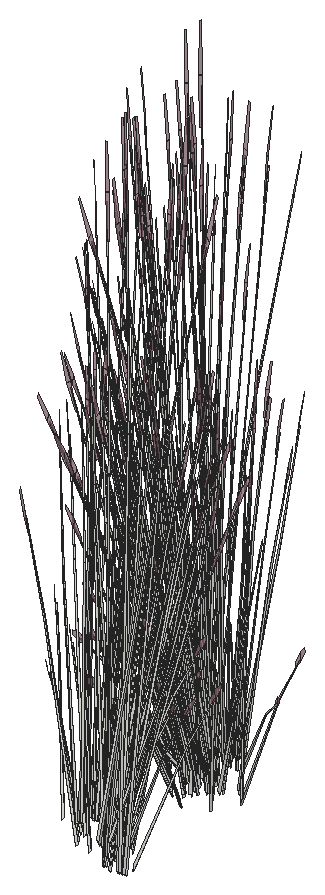
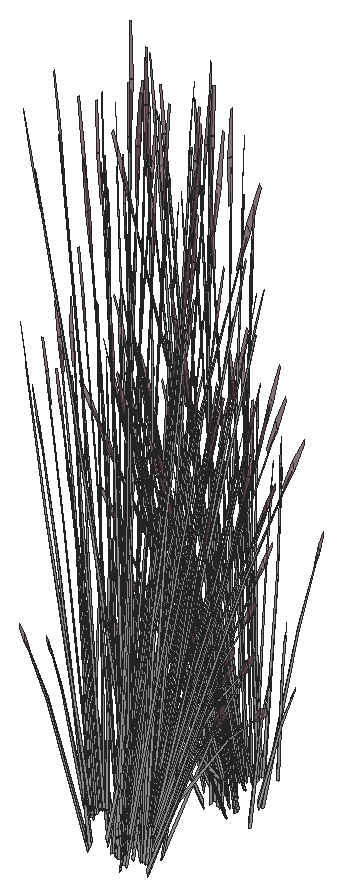
# SketchUp Ruby script. Lengths in inches.
U = 1.inch
M = Sketchup.active_model
def pt(a) = Geom::Point3d.new(a.map { |v| v * U })
def face(e, loops, mat)
  f = e.add_face(loops[0].map { |a| pt(a) })
  loops[1..].each { |l| e.add_face(l.map { |a| pt(a) }).erase! }
  f.material = f.back_material = mat if mat
  f
end
# faces: each face lists its corners as indices into pts; further lists are holes
def faces(e, pts, list, mat = nil) = list.each { |f| face(e, (f[0].is_a?(Array) ? f : [f]).map { |l| l.map { |i| pts[i] } }, mat) }
# xy, xz, yz: faces in a plane at the given z, y or x. An outline is a flat list of corners, or four numbers for a rectangle; further outlines are holes
def ring(l) = l.size == 4 ? [[l[0], l[1]], [l[2], l[1]], [l[2], l[3]], [l[0], l[3]]] : l.each_slice(2).to_a
def flat(e, list, mat, &to3) = list.each { |f| face(e, (f[0].is_a?(Array) ? f : [f]).map { |l| ring(l).map { |u, v| to3.(u, v) } }, mat) }
def xy(e, z, list, mat = nil) = flat(e, list, mat) { |x, y| [x, y, z] }
def xz(e, y, list, mat = nil) = flat(e, list, mat) { |x, z| [x, y, z] }
def yz(e, x, list, mat = nil) = flat(e, list, mat) { |y, z| [x, y, z] }
def lines(e, pts, list) = list.each { |a, b| e.add_line(pt(pts[a]), pt(pts[b])) }
# prism: a flat outline (further loops are holes) pulled along v
def prism(e, loops, v, mat = nil)
  f = face(e, loops, mat); d = Geom::Vector3d.new(v.map { |x| x * U })
  f.pushpull(f.normal.samedirection?(d) ? d.length : -d.length)
end
def box(e, o, s, mat = nil) = prism(e, [[o, [o[0] + s[0], o[1], o[2]], [o[0] + s[0], o[1] + s[1], o[2]], [o[0], o[1] + s[1], o[2]]]], [0, 0, s[2]], mat)
def at(x, y, z, deg = 0) = Geom::Transformation.translation(pt([x, y, z])) * Geom::Transformation.rotation(ORIGIN, Z_AXIS, deg.degrees)
def axes(o, x, y, z) = Geom::Transformation.new([*x, 0, *y, 0, *z, 0, *pt(o).to_a, 1])
def part(name) = M.definitions.add(name)
# library, detail: a bought-in or finely detailed component or shape, given as its bounding box
def library(name, o, s) = part(name).tap { |d| box(d.entities, o, s) }
def detail(e, o, s) = box(e.add_group.entities, o, s)
def put(e, d, t, mat = nil) = e.add_instance(d, t).tap { |i| i.material = mat if mat }
def group(e, t, mat = nil) = e.add_group.tap { |g| g.transformation = t; g.material = mat if mat }.entities
root = M.entities
M.materials.add("LightPink_Translucent").color = [144, 107, 117]
M.materials["LightPink_Translucent"].alpha = 0.75
c1 = part("blade")
p = [[2.15,0.21,22],[0,0.17,0],[0.09,0.45,0],[2.18,0.31,22],[2.29,0.31,22],[0.38,0.45,0],
  [2.48,0.24,33],[2.49,0.24,33],[2.48,0.22,33]]
faces(c1.entities,p,[[0,1,2,3],[4,5,2,3],[6,3,4,7],[8,0,3,6]])
c2 = part("seeds")
p = [[0.3,-0.1,1.38],[-0.01,-0.03,1.59],[-0.01,-0.03,0.03],[0.14,-0.07,-0.07],[0.29,-0.03,3],[0.15,0.01,3.11]]
faces(c2.entities,p,[[0,1,2,3],[1,0,4,5]],"LightPink_Translucent")
c3 = part("blade with seeds")
put(c3.entities,c1,at(0,0,0))
put(c3.entities,c2,axes([2.4,0.25,30.99],[1.5799,-0.05474,1.17369],[-0.12525,1.92788,0.29478],[-0.07173,-0.02425,1.56792]))
put(root,c3,axes([417.64,637.87,155.99],[-0.38233,-0.1167,-0.2617],[0.09626,-0.41098,0.2617],[-0.07708,0.04739,1.17405]))
put(root,c3,axes([414.88,637.03,156.46],[0.14242,0.03872,1.20808],[0.09179,0.39548,-0.25981],[-0.19345,0.07403,0.51652]))
put(root,c3,axes([415.52,636.71,158.54],[0.35672,-0.06741,0.29918],[0.09419,0.38534,-0.38624],[-0.10222,0.1035,0.73904]))
put(root,c3,axes([419.12,636.3,156.28],[0.51243,0,0],[0,0.52715,-0.43598],[0,0.12006,1.38303]))
put(root,c3,axes([414.14,636.54,158.25],[0.0523,0.01265,1.49853],[0.16179,0.41674,-0.1416],[-0.10706,0.10938,0.26519]))
put(root,c3,axes([418.91,636.57,156.13],[-0.51218,-0.00377,-0.04204],[0,-0.52715,0.42192],[-0.0161,0.12,1.33776]))
put(root,c3,axes([417.8,636.11,156.53],[0.46151,0.22505,-0.2458],[-0.22222,0.475,-0.42242],[0.0145,0.11662,1.34921]))
put(root,c3,axes([414.58,637.86,156.61],[0.17079,-0.21377,0.97034],[0.06739,0.33841,0.71294],[-0.12342,0.0606,0.21373]))
put(root,c3,axes([418.69,637.47,158.1],[0.23317,0.29531,-0.29918],[-0.26625,0.27955,0.38624],[0.13527,0.04253,0.73904]))
put(root,c3,axes([418.8,636.65,155.99],[-0.28606,0.29428,-0.2617],[-0.28606,-0.29428,0.2617],[0,0.09479,1.17405]))
put(root,c3,axes([417.57,636.68,156.53],[0.04775,0.53819,-0.2458],[-0.49736,0.03254,-0.42242],[-0.08758,0.07169,1.34921]))
put(root,c3,axes([418.57,637.58,158.27],[-0.02064,0.35866,0.05432],[-0.3116,-0.00983,0.42765],[0.11936,0.03753,0.65209]))
put(root,c3,axes([417.75,636.47,156.14],[-0.19883,0.425,-0.37796],[-0.41314,-0.20454,0.1819],[0,0.09797,1.2135]))
put(root,c3,axes([415.23,636.9375,158.1],[-0.35672,0.06741,-0.29918],[-0.09419,-0.38534,0.38624],[-0.10222,0.1035,0.73904]))
put(root,c3,axes([418.6,637.47,158.27],[-0.30217,0.31079,0.40553],[-0.2606,-0.33005,0.33437],[0.14177,0.05733,0.83914]))
put(root,c3,axes([414.71,637.8,159.05],[0.36162,0.1259,-0.05481],[-0.11124,0.3875,-0.2485],[-0.05915,0.05883,0.81966]))
put(root,c3,axes([417.27,637.09,156.02],[-0.27603,0.35451,-0.52676],[-0.34289,-0.32147,-0.13825],[-0.11061,0.08844,1.16273]))
put(root,c3,axes([417.64,637.83,158.54],[-0.06329,-0.37991,0.29918],[0.36182,-0.10032,-0.38624],[0.09718,0.10887,0.73904]))
put(root,c3,axes([417.76,637.68,156.24],[0.51304,0.1533,0.25983],[-0.12835,0.54797,-0.30828],[-0.08491,0.06858,1.39295]))
put(root,c3,axes([417.73,638.05,155.98],[-0.38354,0.23583,-0.41945],[-0.22925,-0.42288,0],[-0.08735,0.05371,1.33059]))
put(root,c3,axes([419,636.66,155.98],[0,0.47166,-0.41945],[-0.45849,0,0],[0,0.10742,1.33059]))
put(root,c3,axes([417.86,636.71,157.55],[-0.15222,-0.08126,1.44779],[0.31502,-0.34091,0.11706],[0.19634,0.15379,0.61892]))
put(root,c3,axes([417.88,635.64,158.06],[-0.35411,-0.24507,1.16821],[0.37391,-0.38156,0.50405],[0.11425,0.22994,1.12919]))
put(root,c3,axes([415.33,636.68,158.53],[0.37908,0.26007,-0.10273],[-0.21839,0.37663,-0.57019],[-0.1071,0.13092,0.8664]))
put(root,c3,axes([418.42,637.64,156.61],[-0.23074,-0.13562,0.97034],[0.29794,-0.1378,0.71294],[0.08036,0.11673,0.21373]))
put(root,c3,axes([417.61,638.02,158.53],[0.2442,-0.40372,-0.10273],[0.35364,0.23259,-0.57019],[0.12293,0.11406,0.8664]))
put(root,c3,axes([415.84,636.56,157.55],[0.10236,-0.14492,1.44779],[0.25844,0.39118,0.11706],[-0.17726,0.17814,0.61892]))
put(root,c3,axes([415.52,636.98,158.23],[0.10528,0.43067,-0.43168],[-0.39868,0.07534,-0.33437],[-0.11425,0.11568,0.82598]))
put(root,c3,axes([416,637.48,158.54],[0.27728,-0.24833,0.29918],[0.26248,0.28355,-0.38624],[-0.03994,0.14407,0.73904]))
put(root,c3,axes([418.08,637.98,156.28],[0.25622,0.47263,0],[-0.42866,0.26357,-0.43598],[-0.09763,0.06003,1.38303]))
put(root,c3,axes([417.29,638.36,158.25],[0.00121,-0.0571,1.49853],[0.35119,-0.25193,-0.1416],[0.12199,0.08992,0.26519]))
put(root,c3,axes([418.48,638.14,155.54],[0.02986,-0.06809,1.48974],[0.37589,-0.20055,-0.22758],[0.11396,0.1038,0.25375]))
put(root,c3,axes([417.86,636.11,156.68],[-0.01119,-0.44408,1.19347],[0.50665,0.11511,0.50532],[-0.11983,0.243,1.12654]))
put(root,c3,axes([417.99,636.59,156.05],[0.15027,0.43184,-0.5847],[-0.43285,0.15553,-0.15346],[0.01661,0.14623,1.29063]))
put(root,c3,axes([415.75,637.7,158.27],[-0.33677,-0.02198,0.05432],[0.00923,-0.33185,0.42765],[-0.03524,0.12712,0.65209]))
put(root,c3,axes([415.03,638.08,155.54],[0.05497,0.04712,1.48974],[0.09321,0.43661,-0.22758],[-0.12183,0.0931,0.25375]))
put(root,c3,axes([415.85,637.73,158.27],[-0.29182,-0.32181,0.40553],[0.3099,-0.27755,0.33437],[-0.05383,0.15098,0.83914]))
put(root,c3,axes([417.9,637.82,158.23],[0.40438,-0.11212,-0.43168],[0.07074,0.4246,-0.33437],[0.10862,0.12168,0.82598]))
put(root,c3,axes([416.78,637.89,158.54],[0.12355,-0.36271,0.29918],[0.36044,0.10579,-0.38624],[0.03305,0.14603,0.73904]))
put(root,c3,axes([418.46,638.25,156.53],[-0.26279,-0.01479,0.88755],[0.17355,-0.31417,0.49003],[0.10382,0.11162,0.6962]))
put(root,c3,axes([417.7,638.17,158.27],[-0.18625,0.29962,0.05432],[-0.26523,-0.17444,0.42765],[0.08575,0.09606,0.65209]))
put(root,c3,axes([417.26,639.18,159.05],[0.28319,-0.27058,-0.05481],[0.25948,0.29635,-0.2485],[0.01827,0.08397,0.81966]))
put(root,c3,axes([417.78,638.09,158.27],[-0.4076,0.10824,0.40553],[-0.07074,-0.4246,0.33437],[0.09586,0.12514,0.83914]))
put(root,c3,axes([415.77,636.92,157.55],[0.0763,-0.16212,1.44779],[0.3201,0.3355,0.11706],[-0.1444,0.2091,0.61892]))
put(root,c3,axes([417.6,637.49,156.46],[0.00723,-0.15635,1.20808],[0.34559,-0.17464,-0.25981],[0.10668,0.18713,0.51652]))
put(root,c3,axes([416.66,638.22,158.27],[-0.30197,0.1603,0.05432],[-0.1478,-0.29231,0.42765],[0.02916,0.12885,0.65209]))
put(root,c3,axes([415.85,637.83,158.1],[-0.27728,0.24833,-0.29918],[-0.26248,-0.28355,0.38624],[-0.03994,0.14407,0.73904]))
put(root,c3,axes([414.9,637.76,158.26],[-0.01019,0.09334,1.47793],[0.28908,0.3247,-0.23373],[-0.07568,0.15355,0.11853]))
put(root,c3,axes([415.82,637.55,158.84],[0.45039,0.02337,-0.11403],[-0.01231,0.44247,-0.63292],[-0.03129,0.17041,0.9617]))
put(root,c3,axes([416.66,638.04,158.53],[0.40102,-0.2196,-0.10273],[0.19707,0.38974,-0.57019],[0.05291,0.16424,0.8664]))
put(root,c3,axes([416.77,638.18,158.55],[-0.4038,-0.12331,0.45013],[0.13808,-0.40538,0.37115],[0.02427,0.15942,0.93144]))
put(root,c3,axes([416.03,638.8,156.61],[-0.01061,-0.28045,0.97034],[0.26501,0.20003,0.71294],[-0.05212,0.13367,0.21373]))
put(root,c3,axes([416.73,638.125,155.54],[0.06632,-0.02567,1.48974],[0.39894,0.14126,-0.22758],[0.01167,0.15921,0.25375]))
put(root,c3,axes([416.13,637.71,158.5],[0.29336,0.31691,-0.47917],[-0.3099,0.27755,-0.37115],[-0.04464,0.16102,0.91684]))
put(root,c3,axes([415.8125,638.1875,156.66],[0.37228,-0.08352,0.05498],[0.08559,0.3365,-0.7291],[-0.0236,0.17034,0.65354]))
put(root,c3,axes([417,638.02,158.23],[0.40284,0.11824,-0.43168],[-0.13808,0.40538,-0.33437],[0.03694,0.16321,0.82598]))
put(root,c3,axes([417.23,637.18,157.55],[-0.09368,-0.15143,1.44779],[0.43286,-0.12749,0.11706],[0.09783,0.23774,0.61892]))
put(root,c3,axes([416.82,638.27,158.1],[-0.12355,0.36271,-0.29918],[-0.36044,-0.10579,0.38624],[0.03305,0.14603,0.73904]))
put(root,c3,axes([416.04,637.57,158.79],[-0.01066,0.43628,-0.66621],[-0.44902,-0.0293,0.0804],[-0.04739,0.18483,0.94242]))
put(root,c3,axes([414.87,638.71,158.25],[0.04649,-0.02848,1.49853],[0.38427,0.18941,-0.1416],[-0.00903,0.15771,0.26519]))
put(root,c3,axes([416.2,645.72,158.45],[0.09368,0.15143,1.44779],[-0.43286,0.12749,0.11706],[-0.09783,-0.23774,0.61892]))
put(root,c3,axes([416.46,637.26,157.55],[-0.01003,-0.18103,1.44779],[0.43473,0.12009,0.11706],[-0.02689,0.25798,0.61892]))
put(root,c3,axes([416.91,644.72,159.16],[-0.06268,-0.06613,1.47793],[-0.4183,0.04193,-0.23373],[-0.06676,-0.15817,0.11853]))
put(root,c3,axes([417.88,645.5,157.37],[-0.11649,0.09547,1.20808],[-0.34886,-0.1671,-0.25981],[0.06467,-0.20781,0.51652]))
put(root,c3,axes([417.35,645.83,159.39],[-0.19559,-0.38351,-0.60019],[0.40262,-0.21373,0.07243],[-0.04574,-0.1853,0.84903]))
put(root,c3,axes([416.85,637.94,158.48],[0.19559,0.38351,-0.60019],[-0.40262,0.21373,0.07243],[0.04574,0.1853,0.84903]))
put(root,c3,axes([416.08,645.32,157.37],[-0.02482,0.15429,1.20808],[-0.36278,0.12916,-0.25981],[-0.0848,-0.19943,0.51652]))
put(root,c3,axes([415.72,638.55,156.46],[0.12932,-0.07441,1.20808],[0.31929,0.22435,-0.25981],[-0.09503,0.19413,0.51652]))
put(root,c3,axes([416.5625,638.91,158.26],[0.05195,0.07595,1.47793],[0.41921,0.02984,-0.23373],[0.04216,0.1675,0.11853]))
put(root,c3,axes([417.02,644.98,156.44],[-0.06874,0.01699,1.48974],[-0.38012,-0.19128,-0.22758],[0.00638,-0.15955,0.25375]))
put(root,c3,axes([418.17,646.21,159.39],[0.01066,-0.43628,-0.60019],[0.44902,0.0293,0.07243],[0.04739,-0.18483,0.84903]))
put(root,c3,axes([418.79,645.53,159.16],[-0.00396,-0.09387,1.47793],[-0.33411,-0.2713,-0.23373],[0.05166,-0.16446,0.11853]))
put(root,c3,axes([417.39,645.51,159],[0.12355,-0.36271,-0.29918],[0.36044,0.10579,0.38624],[-0.03305,-0.14603,0.73904]))
put(root,c3,axes([417.66,645.99,158.45],[-0.0763,0.16212,1.44779],[-0.3201,-0.3355,0.11706],[0.1444,-0.2091,0.61892]))
put(root,c3,axes([418.7,645.19,159.16],[-0.04162,0.03603,1.49853],[-0.40776,-0.12155,-0.1416],[-0.01476,-0.15722,0.26519]))
put(root,c3,axes([417.21,645.76,159.13],[-0.40284,-0.11824,-0.43168],[0.13808,-0.40538,-0.33437],[-0.03694,-0.16321,0.82598]))
put(root,c3,axes([415.89,638.18,157.12],[0.009,-0.24349,1.30391],[0.40497,0.12861,0.18019],[-0.03509,0.2595,0.61571]))
put(root,c3,axes([417.46,644.74,157.51],[0.05257,0.27504,0.97034],[-0.29163,-0.15233,0.71294],[0.03138,-0.14083,0.21373]))
put(root,c3,axes([418.08,646.06,159.13],[-0.29336,-0.31691,-0.43168],[0.3099,-0.27755,-0.33437],[0.04464,-0.16102,0.82598]))
put(root,c3,axes([416.49,644.5,159.16],[-0.00765,0.05653,1.49853],[-0.37706,0.20517,-0.1416],[-0.11096,-0.10488,0.26519]))
put(root,c3,axes([416.4,645.5,159.48],[0.45651,-0.12123,0.45419],[0.07923,0.47555,0.3745],[-0.10736,-0.14016,0.93983]))
put(root,c3,axes([417.43,645.59,159.18],[0.4038,0.12331,0.40553],[-0.13808,0.40538,0.33437],[-0.02427,-0.15942,0.83914]))
put(root,c3,axes([417.55,645.74,159.43],[-0.40102,0.2196,-0.10273],[-0.19707,-0.38974,-0.57019],[-0.05291,-0.16424,0.8664]))
put(root,c3,axes([418.38,646.23,159.43],[-0.45039,-0.02337,-0.10273],[0.01231,-0.44247,-0.57019],[0.03129,-0.17041,0.8664]))
put(root,c3,axes([418.35,645.95,159],[0.27728,-0.24833,-0.29918],[0.26248,0.28355,0.38624],[0.03994,-0.14407,0.73904]))
put(root,c3,axes([415.96,645.07,157.51],[0.21377,0.16416,0.97034],[-0.31132,0.09868,0.71294],[-0.06661,-0.12616,0.21373]))
put(root,c3,axes([417.54,645.5625,159.17],[0.30197,-0.1603,0.05432],[0.1478,0.29231,0.42765],[-0.02916,-0.12885,0.65209]))
put(root,c3,axes([416.47,645.94,159.39],[-0.34944,-0.22798,-0.60019],[0.24834,-0.39949,0.07243],[-0.1266,-0.13612,0.84903]))
put(root,c3,axes([416.35,645.64,159],[-0.06329,-0.37991,-0.29918],[0.36182,-0.10032,0.38624],[-0.09718,-0.10887,0.73904]))
put(root,c3,axes([416.51,645.61,159.17],[0.18625,-0.29962,0.05432],[0.26523,0.17444,0.42765],[-0.08575,-0.09606,0.65209]))
put(root,c3,axes([415.79,645.57,156.44],[-0.0397,0.06213,1.48974],[-0.40116,0.13396,-0.22758],[-0.09691,-0.12186,0.25375]))
put(root,c3,axes([416.45,647.28,156.95],[-0.1683,-0.48366,-0.58997],[0.48479,-0.17419,-0.15484],[-0.0186,-0.16378,1.30225]))
put(root,c3,axes([415.57,646.19,158.45],[0.15222,0.08126,1.44779],[-0.31502,0.34091,0.11706],[-0.19634,-0.15379,0.61892]))
put(root,c3,axes([418.7,645.8,156.44],[-0.06134,-0.03716,1.48974],[-0.15755,-0.41512,-0.22758],[0.10629,-0.11265,0.25375]))
put(root,c3,axes([417.43,645.89,159.45],[-0.12355,0.36271,0.29918],[-0.36044,-0.10579,-0.38624],[-0.03305,-0.14603,0.73904]))
put(root,c3,axes([416.31,645.96,159.13],[-0.40438,0.11212,-0.43168],[-0.07074,-0.4246,-0.33437],[-0.10862,-0.12168,0.82598]))
put(root,c3,axes([418.35,646.04,159.18],[0.29182,0.32181,0.40553],[-0.3099,0.27755,0.33437],[0.05383,-0.15098,0.83914]))
put(root,c3,axes([416.59,645.58,159.77],[-0.2735,0.45217,-0.11506],[-0.39608,-0.2605,-0.63862],[-0.13768,-0.12775,0.97037]))
put(root,c3,axes([418.46,646.07,159.17],[0.33677,0.02198,0.05432],[-0.00923,0.33185,0.42765],[0.03524,-0.12712,0.65209]))
put(root,c3,axes([418.21,646.3,159.45],[-0.27728,0.24833,0.29918],[-0.26248,-0.28355,-0.38624],[0.03994,-0.14407,0.73904]))
put(root,c3,axes([418.7,646.97,159.39],[0.21406,-0.37215,-0.60019],[0.37511,0.26448,0.07243],[0.12781,-0.13483,0.84903]))
put(root,c3,axes([416.38,645.88,157.18],[-0.25622,-0.47263,0],[0.42866,-0.26357,-0.43598],[0.09763,-0.06003,1.38303]))
put(root,c3,axes([418.6875,646.79,159.13],[-0.10528,-0.43067,-0.43168],[0.39868,-0.07534,-0.33437],[0.11425,-0.11568,0.82598]))
put(root,c3,axes([416.95,645.32,156.98],[-0.28319,0.27058,-0.03288],[-0.25948,-0.29635,-0.1491],[-0.01827,-0.08397,0.4918]))
put(root,c3,axes([415.54,645.45,159.16],[-0.08817,-0.00333,1.47793],[-0.28072,0.33293,-0.23373],[-0.14978,-0.06803,0.11853]))
put(root,c3,axes([418.875,647.1,159.43],[-0.37908,-0.26007,-0.10273],[0.21839,-0.37663,-0.57019],[0.1071,-0.13092,0.8664]))
put(root,c3,axes([417.31,648.52,157.99],[0.35414,0.19019,1.27785],[-0.34693,0.40974,0.50532],[-0.1554,-0.24285,1.07126]))
put(root,c3,axes([416.56,645.95,159.45],[0.06329,0.37991,0.29918],[-0.36182,0.10032,-0.38624],[-0.09718,-0.10887,0.73904]))
put(root,c3,axes([415.46,647.21,156.88],[0,-0.47166,-0.41945],[0.45849,0,0],[0,-0.10742,1.33059]))
put(root,c3,axes([416.73,645.8125,156.88],[0.38354,-0.23583,-0.41945],[0.22925,0.42288,0],[0.08735,-0.05371,1.33059]))
put(root,c3,axes([419.01,646.625,157.37],[-0.1464,-0.01397,1.20808],[-0.14998,-0.37477,-0.25981],[0.17985,-0.10602,0.51652]))
put(root,c3,axes([415.48,646.2,159.48],[0.33843,-0.34808,0.45419],[0.29188,0.36965,0.3745],[-0.15878,-0.06421,0.93983]))
put(root,c3,axes([419.81,646.99,159.16],[-0.05353,-0.00358,1.49853],[-0.22227,-0.38383,-0.1416],[0.08926,-0.1262,0.26519]))
put(root,c3,axes([417.19,646.78,156.92],[0.27603,-0.35451,-0.52676],[0.34289,0.32147,-0.13825],[0.11061,-0.08844,1.16273]))
put(root,c3,axes([419.18,645.9375,157.51],[-0.1365,0.2401,0.97034],[-0.11733,-0.32258,0.71294],[0.11274,-0.08083,0.21373]))
put(root,c3,axes([418.98,646.84,159],[0.35672,-0.06741,-0.29918],[0.09419,0.38534,0.38624],[0.10222,-0.1035,0.73904]))
put(root,c3,axes([415.63,646.2,159.17],[0.02064,-0.35866,0.05432],[0.3116,0.00983,0.42765],[-0.11936,-0.03753,0.65209]))
put(root,c3,axes([416.7,647.4,157.05],[0.19883,-0.425,-0.37796],[0.41314,0.20454,0.1819],[0,-0.09797,1.2135]))
put(root,c3,axes([415.51,646.31,159],[-0.23317,-0.29531,-0.29918],[0.26625,-0.27955,0.38624],[-0.13527,-0.04253,0.73904]))
put(root,c3,axes([416.89,647.19,157.43],[-0.04775,-0.53819,-0.2458],[0.49736,-0.03254,-0.42242],[0.08758,-0.07169,1.34921]))
put(root,c3,axes([415.65,647.22,156.89],[0.28606,-0.29428,-0.2617],[0.28606,0.29428,0.2617],[0,-0.09479,1.17405]))
put(root,c3,axes([415.54,645.81,156.98],[-0.11822,0.38513,-0.03288],[-0.36385,-0.11847,-0.1491],[-0.05524,-0.06299,0.4918]))
put(root,c3,axes([418.6875,647.07,159.45],[-0.35672,0.06741,0.29918],[-0.09419,-0.38534,-0.38624],[0.10222,-0.1035,0.73904]))
put(root,c3,axes([416.66,647.75,157.43],[-0.46151,-0.22505,-0.2458],[0.22222,-0.475,-0.42242],[-0.0145,-0.11662,1.34921]))
put(root,c3,axes([415.34,647.57,157.18],[-0.51243,0,0],[0,-0.52715,-0.43598],[0,-0.12006,1.38303]))
put(root,c3,axes([415.43,646.625,157.37],[0.08001,0.13132,1.20808],[-0.18437,0.35694,-0.25981],[-0.18931,-0.08532,0.51652]))
put(root,c3,axes([416.82,646,156.89],[0.38233,0.1167,-0.2617],[-0.09626,0.41098,0.2617],[0.07708,-0.04739,1.17405]))
put(root,c3,axes([415.76,646.51,159.39],[-0.40965,-0.01136,-0.60019],[0.02751,-0.47821,0.07243],[-0.17355,-0.05047,0.84903]))
put(root,c3,axes([419.01,647.01,159.17],[0.28133,0.19836,0.05432],[-0.16379,0.28248,0.42765],[0.0902,-0.09132,0.65209]))
put(root,c3,axes([418.93,646.92,159.18],[0.10163,0.43409,0.40553],[-0.39868,0.07534,0.33437],[0.1175,-0.10209,0.83914]))
put(root,c3,axes([420.01,647.45,159.16],[0.05687,-0.07184,1.47793],[-0.07279,-0.44069,-0.23373],[0.14268,-0.08356,0.11853]))
put(root,c3,axes([415.74,647.43,157.15],[-0.38118,0.39654,0.25983],[-0.38142,-0.39237,-0.30828],[-0.01331,-0.11261,1.39295]))
put(root,c3,axes([415.2,645.73,159.16],[0.03038,0.04707,1.49853],[-0.14646,0.42312,-0.1416],[-0.14833,0.00306,0.26519]))
put(root,c3,axes([416.95,647.61,157.23],[0.46174,0.2286,0.2033],[-0.22222,0.475,0.42242],[0,-0.1095,1.35626]))
put(root,c3,axes([416.77,648.25,157.24],[0.10862,-0.55889,-0.19793],[0.515,0.09742,0.43313],[-0.08999,-0.07718,1.32161]))
put(root,c3,axes([415.625,646.6,159.13],[-0.29757,0.31243,-0.43168],[-0.2606,-0.33005,-0.33437],[-0.15119,-0.04754,0.82598]))
put(root,c3,axes([415.84,646.46,159.45],[0.23317,0.29531,0.29918],[-0.26625,0.27955,-0.38624],[-0.13527,-0.04253,0.73904]))
put(root,c3,axes([414.95,647.02,157.51],[0.26163,-0.03375,0.97034],[-0.16596,0.29737,0.71294],[-0.12929,-0.04461,0.21373]))
put(root,c3,axes([416.8,647.29,157.48],[-0.44501,0.02912,0.37796],[-0.04024,-0.48332,-0.1819],[0.07967,-0.04899,1.2135]))
put(root,c3,axes([415.78,646.28,159.43],[-0.02194,0.47967,-0.10273],[-0.41546,-0.01311,-0.57019],[-0.16001,-0.03332,0.8664]))
put(root,c3,axes([415.65,647.65,157.27],[0,0.47166,0.41945],[-0.45849,0,0],[0,-0.10742,1.33059]))
put(root,c3,axes([418.89,648.12,159.43],[-0.20619,-0.42709,-0.10273],[0.36595,-0.20988,-0.57019],[0.15422,-0.05635,0.8664]))
put(root,c3,axes([418.87,647.75,159.13],[0.11102,-0.42903,-0.43168],[0.38064,0.14706,-0.33437],[0.15325,-0.03934,0.82598]))
put(root,c3,axes([418.27,646,157.1875],[0.25622,-0.47263,0],[0.42866,0.26357,-0.43598],[0.09763,0.06003,1.38303]))
put(root,c3,axes([415.25,646.9375,158.45],[0.16998,-0.01068,1.44779],[-0.11276,0.46299,0.11706],[-0.24224,-0.02864,0.61892]))
put(root,c3,axes([416.74,648.03,157.05],[-0.24618,-0.39589,-0.37796],[0.37289,-0.27878,0.1819],[-0.07967,-0.04899,1.2135]))
put(root,c3,axes([416.79,647.47,157.17],[0.17817,0.52741,0.38653],[-0.50909,0.1834,0.15168],[0.00622,-0.09691,1.34202]))
put(root,c3,axes([419.28,647.87,156.85],[-0.26394,0.0566,1.1961],[-0.04201,-0.45055,0.06846],[0.18486,-0.06819,0.68062]))
put(root,c3,axes([419.76,647.47,157.09],[-0.25407,-0.3016,-0.05481],[0.27826,-0.27635,-0.2485],[0.07884,-0.01946,0.81966]))
put(root,c3,axes([416.7,647.88,157.48],[-0.19883,0.425,0.37796],[-0.41314,-0.20454,-0.1819],[0,-0.09797,1.2135]))
put(root,c3,axes([417.43,647.51,157.04],[0,-0.54574,0],[0.51243,0,0],[0,0,1.51605]))
put(root,c3,axes([418.05,646.25,157.27],[-0.38354,-0.23583,0.41945],[0.22925,-0.42288,0],[0.08735,0.05371,1.33059]))
put(root,c3,axes([418.8,647.91,159.39],[0.3601,-0.20831,-0.60019],[0.20068,0.4288,0.07243],[0.17399,-0.04871,0.84903]))
put(root,c3,axes([416.51,648.18,156.92],[-0.42629,-0.07733,-0.52676],[0.08996,-0.47699,-0.13825],[-0.12722,-0.0578,1.16273]))
put(root,c3,axes([417.18,647.17,157.17],[-0.33979,0.42804,0.38653],[-0.40368,-0.37784,0.15168],[0.08192,-0.04272,1.34202]))
put(root,c3,axes([417.56,647.93,157.12],[-0.38118,-0.40596,-0.0518],[0.38142,-0.40621,0],[-0.01331,-0.01418,1.48322]))
put(root,c3,axes([416.59,646.46,157.27],[-0.11838,0.46875,0.14904],[-0.43321,-0.13265,0.29641],[0.07483,-0.00228,1.35512]))
put(root,c3,axes([418.75,647.99,159.45],[-0.34057,-0.13158,0.29918],[0.09933,-0.38387,-0.38624],[0.13712,-0.0352,0.73904]))
put(root,c3,axes([415.18,647.29,159.18],[0.11578,-0.43006,0.40553],[0.38064,0.14706,0.33437],[-0.14969,0.02584,0.83914]))
put(root,c3,axes([416.42,646.84,156.52],[-0.40337,0.18883,1.08919],[-0.12839,-0.54182,0.42321],[0.24769,0.00901,1.23883]))
put(root,c3,axes([417.5,646.98,157.39],[0.07906,-0.42093,0.12232],[0.38625,0.07307,-0.3493],[0.07029,0.04322,1.07074]))
put(root,c3,axes([415.15,647.17,159.17],[-0.15051,-0.3216,0.05432],[0.27447,-0.15741,0.42765],[-0.12099,0.03106,0.65209]))
put(root,c3,axes([416.83,647.98,157.17],[0.51796,0.09937,0.38653],[-0.10541,0.56124,0.15168],[-0.07569,-0.05419,1.34202]))
put(root,c3,axes([419.57,647.58,156.44],[-0.02142,-0.07161,1.48974],[0.14855,-0.41887,-0.22758],[0.14984,-0.00603,0.25375]))
put(root,c3,axes([415.14,647.5,156.44],[0.01039,0.07433,1.48974],[-0.20952,0.38819,-0.22758],[-0.14882,-0.01957,0.25375]))
put(root,c3,axes([417.33,647.1,157.48],[-0.24618,-0.39589,0.37796],[0.37289,-0.27878,-0.1819],[0.07967,0.04899,1.2135]))
put(root,c3,axes([416.0625,648.9,156.89],[-0.09626,-0.41098,-0.2617],[0.38233,-0.1167,0.2617],[-0.07708,-0.04739,1.17405]))
